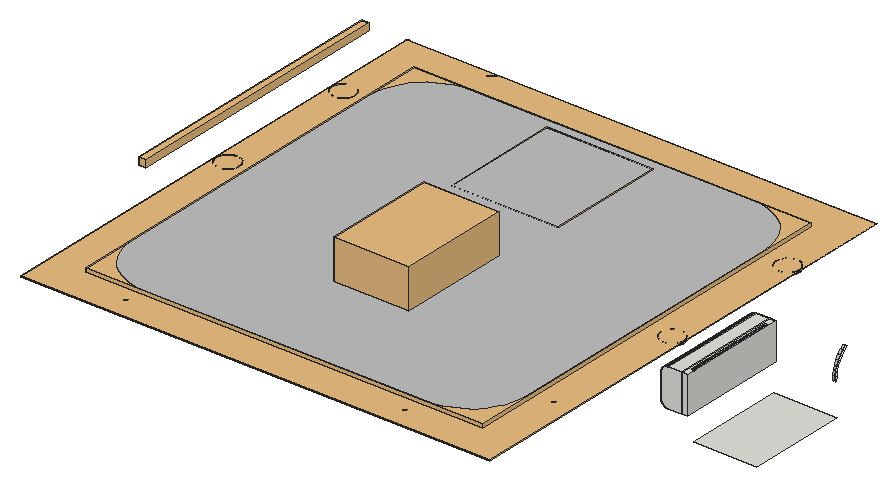
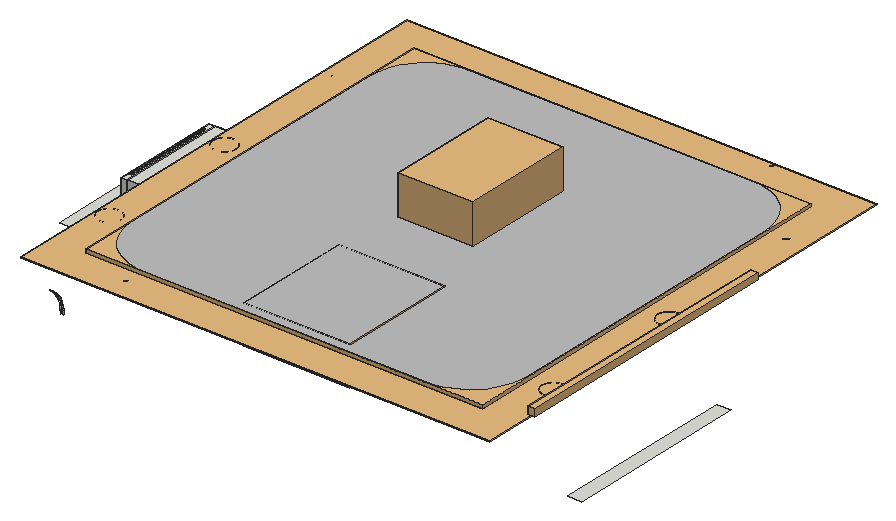
# SketchUp Ruby script. Lengths in inches.
U = 1.inch
M = Sketchup.active_model
def pt(a) = Geom::Point3d.new(a.map { |v| v * U })
def face(e, loops, mat)
  f = e.add_face(loops[0].map { |a| pt(a) })
  loops[1..].each { |l| e.add_face(l.map { |a| pt(a) }).erase! }
  f.material = f.back_material = mat if mat
  f
end
# faces: each face lists its corners as indices into pts; further lists are holes
def faces(e, pts, list, mat = nil) = list.each { |f| face(e, (f[0].is_a?(Array) ? f : [f]).map { |l| l.map { |i| pts[i] } }, mat) }
# xy, xz, yz: faces in a plane at the given z, y or x. An outline is a flat list of corners, or four numbers for a rectangle; further outlines are holes
def ring(l) = l.size == 4 ? [[l[0], l[1]], [l[2], l[1]], [l[2], l[3]], [l[0], l[3]]] : l.each_slice(2).to_a
def flat(e, list, mat, &to3) = list.each { |f| face(e, (f[0].is_a?(Array) ? f : [f]).map { |l| ring(l).map { |u, v| to3.(u, v) } }, mat) }
def xy(e, z, list, mat = nil) = flat(e, list, mat) { |x, y| [x, y, z] }
def xz(e, y, list, mat = nil) = flat(e, list, mat) { |x, z| [x, y, z] }
def yz(e, x, list, mat = nil) = flat(e, list, mat) { |y, z| [x, y, z] }
def lines(e, pts, list) = list.each { |a, b| e.add_line(pt(pts[a]), pt(pts[b])) }
# prism: a flat outline (further loops are holes) pulled along v
def prism(e, loops, v, mat = nil)
  f = face(e, loops, mat); d = Geom::Vector3d.new(v.map { |x| x * U })
  f.pushpull(f.normal.samedirection?(d) ? d.length : -d.length)
end
def box(e, o, s, mat = nil) = prism(e, [[o, [o[0] + s[0], o[1], o[2]], [o[0] + s[0], o[1] + s[1], o[2]], [o[0], o[1] + s[1], o[2]]]], [0, 0, s[2]], mat)
def at(x, y, z, deg = 0) = Geom::Transformation.translation(pt([x, y, z])) * Geom::Transformation.rotation(ORIGIN, Z_AXIS, deg.degrees)
def axes(o, x, y, z) = Geom::Transformation.new([*x, 0, *y, 0, *z, 0, *pt(o).to_a, 1])
def part(name) = M.definitions.add(name)
# library, detail: a bought-in or finely detailed component or shape, given as its bounding box
def library(name, o, s) = part(name).tap { |d| box(d.entities, o, s) }
def detail(e, o, s) = box(e.add_group.entities, o, s)
def put(e, d, t, mat = nil) = e.add_instance(d, t).tap { |i| i.material = mat if mat }
def group(e, t, mat = nil) = e.add_group.tap { |g| g.transformation = t; g.material = mat if mat }.entities
root = M.entities
M.materials.add("[0131_Silver]1").color = [192, 192, 192]
M.materials.add("[Color_004]").color = [142, 142, 142]
M.materials.add("[Color_007]").color = [58, 58, 58]
M.materials.add("[Color_C12]").color = [153, 91, 30]
M.materials.add("[Polished Concrete New]").color = [200, 200, 203]
c1 = library("elliptical+hanging+lamp",[-24.47,-37.92,-16.02],[48.84,73.52,59.72])
c2 = library("Group\#200",[-80.34,-149.03,-93.91],[1.18,2.79,3])
c3 = library("Group\#201",[-80.34,-139.83,-93.89],[1.18,2.84,2.98])
c4 = library("Group\#226",[-0.5,-0.5,0],[173.13,179.13,1.53])
c5 = library("Mesh Light\#5",[-0.5,-0.5,-0.1],[1,1,0.2])
c6 = library("Group\#190",[-80.46,-65.36,-92.6],[1.38,3.58,3.59])
c7 = library("Group\#194",[-88.79,0.67,-41.3125],[0.99,6.14,4.87])
c8 = library("Group\#191",[-88.79,21.34,-41.3125],[0.99,6.53,4.87])
c9 = library("Component\#44",[-0.76,-0.76,-71.54],[3.88,3.88,152.54])
c10 = library("031_FANZART_Zen",[-27.59,-27.12,5.07],[46.53,51.77,17.09])
xy(root,122.28,[[234,631.3,261.625,675.05]])
xy(root,123.47,[[0,635.77,6,717.2]])
xy(root,155.19,[[57.9375,551,54.8,551.2,51.72,551.82,48.75,552.83,45.9375,554.21,43.33,555.96,40.97,558.03,38.9,560.39,37.15,563,35.76,565.8125,34.75,568.79,34.14,571.87,33.9375,575,33.9375,705.125,34.14,708.26,34.75,711.34,35.76,714.3125,37.15,717.125,38.9,719.74,40.97,722.1,43.33,724.17,45.9375,725.91,48.75,727.3,51.72,728.31,54.8,728.92,57.9375,729.125,182.0625,729.125,185.2,728.92,188.28,728.31,191.25,727.3,194.0625,725.91,196.67,724.17,199.03,722.1,201.1,719.74,202.85,717.125,204.24,714.3125,205.25,711.34,205.86,708.26,206.0625,705.125,206.0625,575,205.86,571.87,205.25,568.79,204.24,565.8125,202.85,563,201.1,560.39,199.03,558.03,196.67,555.96,194.0625,554.21,191.25,552.83,188.28,551.82,185.2,551.2,182.0625,551]],"[0131_Silver]1")
yz(root,33.9375,[[575,152.12,705.125,153.65]])
yz(root,206.0625,[[575,152.12,705.125,153.65]],"[0131_Silver]1")
p = [[232.4375,709.3125,111.52],[233.03,709.3125,111.52],[233.03,709.4375,113.41],[232.4375,709.4375,113.41],[234,709.3125,111.52],[234,709.4375,113.41],
  [233.625,709.4375,113.41],[233.625,709.3125,111.52],[233.03,709.81,115.27],[232.4375,709.81,115.27],[234,709.81,115.27],[233.625,709.81,115.27],
  [233.03,710.42,117.07],[232.4375,710.42,117.07],[234,710.42,117.07],[233.625,710.42,117.07],[233.03,711.26,118.77],[232.4375,711.26,118.77],
  [234,711.26,118.77],[233.625,711.26,118.77],[233.03,712.3125,120.35],[232.4375,712.3125,120.35],[234,712.3125,120.35],[233.625,712.3125,120.35],
  [233.03,713.5625,121.78],[232.4375,713.5625,121.78],[234,713.5625,121.78],[233.625,713.5625,121.78],[233.03,714.99,123.03],[232.4375,714.99,123.03],
  [234,714.99,123.03],[233.625,714.99,123.03],[215.71,580.89,152.12],[217,581.0625,152.12],[217,581.0625,153.31],[215.71,580.89,153.31],
  [218.29,580.89,152.12],[218.29,580.89,153.31],[23,635.91,152.12],[21.71,636.09,152.12],[21.71,636.09,153.44],[23,635.91,153.44],
  [24.29,636.09,152.12],[24.29,636.09,153.44],[217,635.91,152.12],[215.71,636.09,152.12],[215.71,636.09,153.31],[217,635.91,153.31],
  [218.29,636.09,152.12],[218.29,636.09,153.31],[20.5,636.58,152.12],[20.5,636.58,153.44],[25.5,636.58,152.12],[25.5,636.58,153.44],
  [214.5,636.58,152.12],[214.5,636.58,153.31],[219.5,636.58,152.12],[219.5,636.58,153.31],[19.46,637.38,152.12],[19.46,637.38,153.44],
  [26.54,637.38,152.12],[26.54,637.38,153.44],[213.46,637.38,152.12],[213.46,637.38,153.31],[220.54,637.38,152.12],[220.54,637.38,153.31],
  [18.67,638.41,152.12],[18.67,638.41,153.44],[27.33,638.41,152.12],[27.33,638.41,153.44],[212.67,638.41,152.12],[212.67,638.41,153.31],
  [221.33,638.41,152.12],[221.33,638.41,153.31],[18.17,639.62,152.12],[18.17,639.62,153.44],[27.83,639.62,152.12],[27.83,639.62,153.44],
  [212.17,639.62,152.12],[212.17,639.62,153.31],[221.83,639.62,152.12],[221.83,639.62,153.31],[18,640.91,152.12],[18,640.91,153.44],
  [28,640.91,152.12],[28,640.91,153.44],[212,640.91,152.12],[212,640.91,153.31],[222,640.91,152.12],[222,640.91,153.31],
  [18.17,642.21,152.12],[18.17,642.21,153.44],[27.83,642.21,152.12],[27.83,642.21,153.44],[212.17,642.21,152.12],[212.17,642.21,153.31],
  [221.83,642.21,152.12],[221.83,642.21,153.31],[18.67,643.41,152.12],[18.67,643.41,153.44],[27.33,643.41,152.12],[27.33,643.41,153.44],
  [212.67,643.41,152.12],[212.67,643.41,153.31],[221.33,643.41,152.12],[221.33,643.41,153.31],[19.46,644.45,152.12],[19.46,644.45,153.44],
  [26.54,644.45,152.12],[26.54,644.45,153.44],[213.46,644.45,152.12],[213.46,644.45,153.31],[220.54,644.45,152.12],[220.54,644.45,153.31],
  [20.5,645.24,152.12],[20.5,645.24,153.44],[25.5,645.24,152.12],[25.5,645.24,153.44],[214.5,645.24,152.12],[214.5,645.24,153.31],
  [219.5,645.24,152.12],[219.5,645.24,153.31],[21.71,645.74,152.12],[21.71,645.74,153.44],[24.29,645.74,152.12],[24.29,645.74,153.44],
  [215.71,645.74,152.12],[215.71,645.74,153.31],[218.29,645.74,152.12],[218.29,645.74,153.31],[23,645.91,152.12],[23,645.91,153.44],
  [217,645.91,152.12],[217,645.91,153.31],[23,699.0625,152.12],[21.71,699.23,152.12],[21.71,699.23,153.44],[23,699.0625,153.44],
  [24.29,699.23,152.12],[24.29,699.23,153.44],[217,699.0625,152.12],[215.71,699.23,152.12],[215.71,699.23,153.31],[217,699.0625,153.31],
  [218.29,699.23,152.12],[218.29,699.23,153.31],[20.5,699.73,152.12],[20.5,699.73,153.44],[25.5,699.73,152.12],[25.5,699.73,153.44],
  [214.5,699.73,152.12],[214.5,699.73,153.31],[219.5,699.73,152.12],[219.5,699.73,153.31],[19.46,700.53,152.12],[19.46,700.53,153.44],
  [26.54,700.53,152.12],[26.54,700.53,153.44],[213.46,700.53,152.12],[213.46,700.53,153.31],[220.54,700.53,152.12],[220.54,700.53,153.31],
  [18.67,701.5625,152.12],[18.67,701.5625,153.44],[27.33,701.5625,152.12],[27.33,701.5625,153.44],[212.67,701.5625,152.12],[212.67,701.5625,153.31],
  [221.33,701.5625,152.12],[221.33,701.5625,153.31],[18.17,702.77,152.12],[18.17,702.77,153.44],[27.83,702.77,152.12],[27.83,702.77,153.44],
  [212.17,702.77,152.12],[212.17,702.77,153.31],[221.83,702.77,152.12],[221.83,702.77,153.31],[18,704.0625,152.12],[18,704.0625,153.44],
  [28,704.0625,152.12],[28,704.0625,153.44],[212,704.0625,152.12],[212,704.0625,153.31],[222,704.0625,152.12],[222,704.0625,153.31],
  [18.17,705.36,152.12],[18.17,705.36,153.44],[27.83,705.36,152.12],[27.83,705.36,153.44],[212.17,705.36,152.12],[212.17,705.36,153.31],
  [221.83,705.36,152.12],[221.83,705.36,153.31],[34.14,708.26,152.12],[34.14,708.26,153.65],[33.9375,705.125,153.65],[33.9375,705.125,152.12],
  [206.0625,705.125,152.12],[206.0625,705.125,153.65],[205.86,708.26,153.65],[205.86,708.26,152.12],[18.67,706.5625,152.12],[18.67,706.5625,153.44],
  [27.33,706.5625,152.12],[27.33,706.5625,153.44],[212.67,706.5625,152.12],[212.67,706.5625,153.31],[221.33,706.5625,152.12],[221.33,706.5625,153.31],
  [19.46,707.6,152.12],[19.46,707.6,153.44],[26.54,707.6,152.12],[26.54,707.6,153.44],[213.46,707.6,152.12],[213.46,707.6,153.31],
  [220.54,707.6,152.12],[220.54,707.6,153.31],[20.5,708.39,152.12],[20.5,708.39,153.44],[25.5,708.39,152.12],[25.5,708.39,153.44],
  [214.5,708.39,152.12],[214.5,708.39,153.31],[219.5,708.39,152.12],[219.5,708.39,153.31],[34.75,711.34,152.12],[34.75,711.34,153.65],
  [205.25,711.34,153.65],[205.25,711.34,152.12],[21.71,708.89,152.12],[21.71,708.89,153.44],[24.29,708.89,152.12],[24.29,708.89,153.44],
  [215.71,708.89,152.12],[215.71,708.89,153.31],[218.29,708.89,152.12],[218.29,708.89,153.31],[23,709.0625,152.12],[23,709.0625,153.44],
  [217,709.0625,152.12],[217,709.0625,153.31],[35.76,714.3125,152.12],[35.76,714.3125,153.65],[204.24,714.3125,153.65],[204.24,714.3125,152.12]]
faces(root,p,[[0,1,2,3],[3,2,8,9],[9,8,12,13],[13,12,16,17],[17,16,20,21],[21,20,24,25],[25,24,28,29]],"[Polished Concrete New]")
faces(root,p,[[4,5,6,7],[5,10,11,6],[10,14,15,11],[14,18,19,15],[18,22,23,19],[22,26,27,23],[26,30,31,27],[32,33,34,35],
  [33,36,37,34],[38,39,40,41],[42,38,41,43],[44,45,46,47],[48,44,47,49],[39,50,51,40],[52,42,43,53],[45,54,55,46],
  [56,48,49,57],[50,58,59,51],[60,52,53,61],[54,62,63,55],[64,56,57,65],[58,66,67,59],[68,60,61,69],[62,70,71,63],
  [72,64,65,73],[66,74,75,67],[76,68,69,77],[70,78,79,71],[80,72,73,81],[74,82,83,75],[84,76,77,85],[78,86,87,79],
  [88,80,81,89],[82,90,91,83],[92,84,85,93],[86,94,95,87],[96,88,89,97],[90,98,99,91],[100,92,93,101],[94,102,103,95],
  [104,96,97,105],[98,106,107,99],[108,100,101,109],[102,110,111,103],[112,104,105,113],[106,114,115,107],[116,108,109,117],[110,118,119,111],
  [120,112,113,121],[114,122,123,115],[124,116,117,125],[118,126,127,119],[128,120,121,129],[122,130,131,123],[130,124,125,131],[126,132,133,127],
  [132,128,129,133],[134,135,136,137],[138,134,137,139],[140,141,142,143],[144,140,143,145],[135,146,147,136],[148,138,139,149],[141,150,151,142],
  [152,144,145,153],[146,154,155,147],[156,148,149,157],[150,158,159,151],[160,152,153,161],[154,162,163,155],[164,156,157,165],[158,166,167,159],
  [168,160,161,169],[162,170,171,163],[172,164,165,173],[166,174,175,167],[176,168,169,177],[170,178,179,171],[180,172,173,181],[174,182,183,175],
  [184,176,177,185],[178,186,187,179],[188,180,181,189],[182,190,191,183],[192,184,185,193],[194,195,196,197],[186,202,203,187],[204,188,189,205],
  [190,206,207,191],[208,192,193,209],[202,210,211,203],[212,204,205,213],[206,214,215,207],[216,208,209,217],[210,218,219,211],[220,212,213,221],
  [214,222,223,215],[224,216,217,225],[226,227,195,194],[218,230,231,219],[232,220,221,233],[222,234,235,223],[236,224,225,237],[230,238,239,231],
  [238,232,233,239],[234,240,241,235],[240,236,237,241],[242,243,227,226]])
faces(root,p,[[198,199,200,201],[201,200,228,229],[229,228,244,245]],"[0131_Silver]1")
put(root,c1,axes([121.33,621.73,143],[0.67,0,0],[0,0.67,0],[0,0,0.67]))
g1 = group(root,at(233.9,652.1,149.98))
prism(g1,[[[-10.63,-19.85,-11.9],[-10.63,-19.78,-12.29],[-10.63,-19.87,-12.29],[-10.63,-19.93,-11.9]]],[0.16,0,0],"[Color_004]")
g2 = group(root,at(233.9,652.1,149.98))
detail(g2,[-10.63,-19.86,-12.43],[0.15,0.1,0.1])
put(root,c2,axes([233.9,652.1,149.98],[0.13234,0,0],[0,0.13234,0],[0,0,0.13234]))
g3 = group(root,at(233.9,652.1,149.98),"[Color_004]")
prism(g3,[[[-10.63,-19.3,-12.03],[-10.63,-19.16,-12.29],[-10.63,-19.1,-12.03],[-10.63,-19.01,-12.03],[-10.63,-19.09,-12.42],[-10.63,-19.1875,-12.42],[-10.63,-19.4,-12.03]]],[0.16,0,0],"[Color_004]")
g4 = group(root,at(233.9,652.1,149.98))
detail(g4,[-10.63,-19.02,-11.99],[0.15,0.09,0.09])
g5 = group(root,at(233.9,652.1,149.98))
prism(g5,[[[-10.63,-18.93,-12.42],[-10.63,-19,-12.03],[-10.63,-18.92,-12.03],[-10.63,-18.85,-12.42]]],[0.16,0,0],"[Color_004]")
g6 = group(root,at(233.9,652.1,149.98))
detail(g6,[-10.63,-18.86,-12.43],[0.15,0.33,0.53])
put(root,c3,axes([233.9,652.1,149.98],[0.13234,0,0],[0,0.13234,0],[0,0,0.13234]))
put(root,c4,at(33.9375,551,153.65))
g7 = group(root,at(18,535.0625,153.31))
xy(g7,0,[[163,0,161.71,0.17,160.5,0.67,159.46,1.46,158.67,2.5,158.17,3.71,158,5,158.17,6.29,158.67,7.5,159.46,8.54,160.5,9.33,161.71,9.83,163,10,164.29,9.83,165.5,9.33,166.54,8.54,167.33,7.5,167.83,6.29,168,5,167.83,3.71,167.33,2.5,166.54,1.46,165.5,0.67,164.29,0.17],[199,36,197.71,36.17,196.5,36.67,195.46,37.46,194.67,38.5,194.17,39.71,194,41,194.17,42.29,194.67,43.5,195.46,44.54,196.5,45.33,197.71,45.83,199,46,200.29,45.83,201.5,45.33,202.54,44.54,203.33,43.5,203.83,42.29,204,41,203.83,39.71,203.33,38.5,202.54,37.46,201.5,36.67,200.29,36.17],[199,100.85,197.71,101.02,196.5,101.52,195.46,102.32,194.67,103.35,194.17,104.56,194,105.85,194.17,107.15,194.67,108.35,195.46,109.39,196.5,110.18,197.71,110.68,199,110.85,200.29,110.68,201.5,110.18,202.54,109.39,203.33,108.35,203.83,107.15,204,105.85,203.83,104.56,203.33,103.35,202.54,102.32,201.5,101.52,200.29,101.02],[199,164,197.71,164.17,196.5,164.67,195.46,165.46,194.67,166.5,194.17,167.71,194,169,194.17,170.29,194.67,171.5,195.46,172.54,196.5,173.33,197.71,173.83,199,174,200.29,173.83,201.5,173.33,202.54,172.54,203.33,171.5,203.83,170.29,204,169,203.83,167.71,203.33,166.5,202.54,165.46,201.5,164.67,200.29,164.17],[163,200,161.71,200.17,160.5,200.67,159.46,201.46,158.67,202.5,158.17,203.71,158,205,158.17,206.29,158.67,207.5,159.46,208.54,160.5,209.33,161.71,209.83,163,210,164.29,209.83,165.5,209.33,166.54,208.54,167.33,207.5,167.83,206.29,168,205,167.83,203.71,167.33,202.5,166.54,201.46,165.5,200.67,164.29,200.17]])
xy(g7,0.125,[[41,0,39.71,0.17,38.5,0.67,37.46,1.46,36.67,2.5,36.17,3.71,36,5,36.17,6.29,36.67,7.5,37.46,8.54,38.5,9.33,39.71,9.83,41,10,42.29,9.83,43.5,9.33,44.54,8.54,45.33,7.5,45.83,6.29,46,5,45.83,3.71,45.33,2.5,44.54,1.46,43.5,0.67,42.29,0.17],[5,36,3.71,36.17,2.5,36.67,1.46,37.46,0.67,38.5,0.17,39.71,0,41,0.17,42.29,0.67,43.5,1.46,44.54,2.5,45.33,3.71,45.83,5,46,6.29,45.83,7.5,45.33,8.54,44.54,9.33,43.5,9.83,42.29,10,41,9.83,39.71,9.33,38.5,8.54,37.46,7.5,36.67,6.29,36.17],[5,100.85,3.71,101.02,2.5,101.52,1.46,102.32,0.67,103.35,0.17,104.56,0,105.85,0.17,107.15,0.67,108.35,1.46,109.39,2.5,110.18,3.71,110.68,5,110.85,6.29,110.68,7.5,110.18,8.54,109.39,9.33,108.35,9.83,107.15,10,105.85,9.83,104.56,9.33,103.35,8.54,102.32,7.5,101.52,6.29,101.02],[5,164,3.71,164.17,2.5,164.67,1.46,165.46,0.67,166.5,0.17,167.71,0,169,0.17,170.29,0.67,171.5,1.46,172.54,2.5,173.33,3.71,173.83,5,174,6.29,173.83,7.5,173.33,8.54,172.54,9.33,171.5,9.83,170.29,10,169,9.83,167.71,9.33,166.5,8.54,165.46,7.5,164.67,6.29,164.17],[41,200,39.71,200.17,38.5,200.67,37.46,201.46,36.67,202.5,36.17,203.71,36,205,36.17,206.29,36.67,207.5,37.46,208.54,38.5,209.33,39.71,209.83,41,210,42.29,209.83,43.5,209.33,44.54,208.54,45.33,207.5,45.83,206.29,46,205,45.83,203.71,45.33,202.5,44.54,201.46,43.5,200.67,42.29,200.17]])
put(g7,c5,axes([102,105,0.0625],[205,0,0],[0,211,0],[0,0,1.125]))
put(root,c6,axes([233.88,652.1,149.98],[0.13234,0,0],[0,0.13234,0],[0,0,0.13234]))
g8 = group(root,at(234,652.1,149.98))
detail(g8,[-11.75,-3.66,-5.47],[0.13,0.83,0.65])
g9 = group(root,at(234,652.1,149.98),"[Color_004]")
prism(g9,[[[-11.62,-1.84,-5.47],[-11.62,-1.63,-5.47],[-11.62,-1.8,-4.82],[-11.62,-2.07,-4.82],[-11.62,-2.21,-5.26],[-11.62,-2.36,-4.82],[-11.62,-2.62,-4.82],[-11.62,-2.78,-5.47],[-11.62,-2.57,-5.47],[-11.62,-2.46,-5.04],[-11.62,-2.33,-5.47],[-11.62,-2.1,-5.47],[-11.62,-1.96,-5.02]]],[-0.13,0,0],"[Color_004]")
g10 = group(root,at(234,652.1,149.98))
prism(g10,[[[-11.62,-1.05,-5.22],[-11.62,-0.98,-5.07],[-11.62,-1.47,-5.07],[-11.62,-1.58,-5.22]]],[-0.13,0,0],"[Color_004]")
g11 = group(root,at(234,652.1,149.98))
detail(g11,[-11.75,-1.58,-5.47],[0.13,0.83,0.65])
g12 = group(root,at(234,652.1,149.98))
prism(g12,[[[-11.62,0.03,-4.98],[-11.62,0.03,-4.82],[-11.62,-0.69,-4.82],[-11.62,-0.69,-4.98],[-11.62,-0.46,-4.98],[-11.62,-0.46,-5.47],[-11.62,-0.22,-5.47],[-11.62,-0.22,-4.98]]],[-0.13,0,0],"[Color_004]")
g13 = group(root,at(234,652.1,149.98))
xy(g13,-16.31,[[-2.61,-24.02,0,24.02]])
xy(g13,-2.9,[[-1.41,-20.07,-1.09,-15.28],[-0.97,-20.07,-0.65,-15.28],[-0.53,-20.07,-0.22,-15.28],[-1.41,-15.02,-1.09,-10.23],[-0.97,-15.02,-0.65,-10.23],
  [-0.53,-15.02,-0.22,-10.23],[-1.41,-9.97,-1.09,-5.18],[-0.97,-9.97,-0.65,-5.18],[-0.53,-9.97,-0.22,-5.18],[-1.41,-4.92,-1.09,-0.13],
  [-0.97,-4.92,-0.65,-0.13],[-0.53,-4.92,-0.22,-0.13],[-1.41,0.13,-1.09,4.92],[-0.97,0.13,-0.65,4.92],[-0.53,0.13,-0.22,4.92],
  [-1.41,5.18,-1.09,9.97],[-0.97,5.18,-0.65,9.97],[-0.53,5.18,-0.22,9.97],[-1.41,10.23,-1.09,15.02],[-0.97,10.23,-0.65,15.02],
  [-0.53,10.23,-0.22,15.02],[-1.41,15.28,-1.09,20.07],[-0.97,15.28,-0.65,20.07],[-0.53,15.28,-0.22,20.07]])
xy(g13,0,[[[-2.61,-24.02,0,24.02],[-1.41,5.18,-1.41,15.02,-1.09,15.02,-1.09,10.23,-1.41,10.23,-1.41,9.97,-1.09,9.97,-1.09,5.18],[-0.53,5.18,-0.53,9.97,-0.22,9.97,-0.22,10.23,-0.53,10.23,-0.53,15.02,-0.22,15.02,-0.22,5.18],[-0.97,15.28,-0.65,20.07],[-0.53,15.28,-0.22,20.07],[-1.41,15.28,-1.09,20.07],[-1.41,-20.07,-1.09,-15.28],[-0.53,-20.07,-0.22,-15.28],[-0.97,-20.07,-0.65,-15.28],[-0.97,5.18,-0.65,9.97],[-0.53,-9.97,-0.22,-5.18],[-0.97,-9.97,-0.65,-5.18],[-1.41,-9.97,-1.09,-5.18],[-0.97,10.23,-0.65,15.02],[-0.97,0.13,-0.65,4.92],[-0.53,0.13,-0.22,4.92],[-1.41,0.13,-1.09,4.92],[-0.53,-15.02,-0.22,-10.23],[-1.41,-15.02,-1.09,-10.23],[-1.41,-4.92,-1.09,-0.13],[-0.97,-4.92,-0.65,-0.13],[-0.53,-4.92,-0.22,-0.13],[-0.97,-15.02,-0.65,-10.23]]])
xz(g13,-24.02,[[-2.61,-16.31,0,0]])
xz(g13,-20.07,[[-1.41,-2.9,-1.09,0],[-0.97,-2.9,-0.65,0],[-0.53,-2.9,-0.22,0]])
xz(g13,-15.28,[[-1.41,-2.9,-1.09,0],[-0.97,-2.9,-0.65,0],[-0.53,-2.9,-0.22,0]])
xz(g13,-15.02,[[-1.41,-2.9,-1.09,0],[-0.97,-2.9,-0.65,0],[-0.53,-2.9,-0.22,0]])
xz(g13,-10.23,[[-1.41,-2.9,-1.09,0],[-0.97,-2.9,-0.65,0],[-0.53,-2.9,-0.22,0]])
xz(g13,-9.97,[[-1.41,-2.9,-1.09,0],[-0.97,-2.9,-0.65,0],[-0.53,-2.9,-0.22,0]])
xz(g13,-5.18,[[-1.41,-2.9,-1.09,0],[-0.97,-2.9,-0.65,0],[-0.53,-2.9,-0.22,0]])
xz(g13,-4.92,[[-1.41,-2.9,-1.09,0],[-0.97,-2.9,-0.65,0],[-0.53,-2.9,-0.22,0]])
xz(g13,-0.13,[[-1.41,-2.9,-1.09,0],[-0.97,-2.9,-0.65,0],[-0.53,-2.9,-0.22,0]])
xz(g13,0.13,[[-1.41,-2.9,-1.09,0],[-0.97,-2.9,-0.65,0],[-0.53,-2.9,-0.22,0]])
xz(g13,4.92,[[-1.41,-2.9,-1.09,0],[-0.97,-2.9,-0.65,0],[-0.53,-2.9,-0.22,0]])
xz(g13,5.18,[[-1.41,-2.9,-1.09,0],[-0.97,-2.9,-0.65,0],[-0.53,-2.9,-0.22,0]])
xz(g13,9.97,[[-1.41,-2.9,-1.09,0],[-0.97,-2.9,-0.65,0],[-0.53,-2.9,-0.22,0]])
xz(g13,10.23,[[-1.41,-2.9,-1.09,0],[-0.97,-2.9,-0.65,0],[-0.53,-2.9,-0.22,0]])
xz(g13,15.02,[[-1.41,-2.9,-1.09,0],[-0.97,-2.9,-0.65,0],[-0.53,-2.9,-0.22,0]])
xz(g13,15.28,[[-1.41,-2.9,-1.09,0],[-0.97,-2.9,-0.65,0],[-0.53,-2.9,-0.22,0]])
xz(g13,20.07,[[-1.41,-2.9,-1.09,0],[-0.97,-2.9,-0.65,0],[-0.53,-2.9,-0.22,0]])
xz(g13,24.02,[[-2.61,-16.31,0,0]])
yz(g13,-2.61,[[-24.02,-16.31,24.02,0]])
yz(g13,-1.41,[[-20.07,-2.9,-15.28,0],[-15.02,-2.9,-10.23,0],[-9.97,-2.9,-5.18,0],[-4.92,-2.9,-0.13,0],[0.13,-2.9,4.92,0],
  [5.18,-2.9,9.97,0],[10.23,-2.9,15.02,0],[15.28,-2.9,20.07,0]])
yz(g13,-1.09,[[-20.07,-2.9,-15.28,0],[-15.02,-2.9,-10.23,0],[-9.97,-2.9,-5.18,0],[-4.92,-2.9,-0.13,0],[0.13,-2.9,4.92,0],
  [5.18,-2.9,9.97,0],[10.23,-2.9,15.02,0],[15.28,-2.9,20.07,0]])
yz(g13,-0.97,[[-20.07,-2.9,-15.28,0],[-15.02,-2.9,-10.23,0],[-9.97,-2.9,-5.18,0],[-4.92,-2.9,-0.13,0],[0.13,-2.9,4.92,0],
  [5.18,-2.9,9.97,0],[10.23,-2.9,15.02,0],[15.28,-2.9,20.07,0]])
yz(g13,-0.65,[[-20.07,-2.9,-15.28,0],[-15.02,-2.9,-10.23,0],[-9.97,-2.9,-5.18,0],[-4.92,-2.9,-0.13,0],[0.13,-2.9,4.92,0],
  [5.18,-2.9,9.97,0],[10.23,-2.9,15.02,0],[15.28,-2.9,20.07,0]])
yz(g13,-0.53,[[-20.07,-2.9,-15.28,0],[-15.02,-2.9,-10.23,0],[-9.97,-2.9,-5.18,0],[-4.92,-2.9,-0.13,0],[0.13,-2.9,4.92,0],
  [5.18,-2.9,9.97,0],[10.23,-2.9,15.02,0],[15.28,-2.9,20.07,0]])
yz(g13,-0.22,[[-20.07,-2.9,-15.28,0],[-15.02,-2.9,-10.23,0],[-9.97,-2.9,-5.18,0],[-4.92,-2.9,-0.13,0],[0.13,-2.9,4.92,0],
  [5.18,-2.9,9.97,0],[10.23,-2.9,15.02,0],[15.28,-2.9,20.07,0]])
yz(g13,0,[[-24.02,-16.31,24.02,0]])
g14 = group(root,at(234,652.1,149.98))
xy(g14,-16.31,[[-8.49,-24.02,-2.61,-20.33],[-8.49,20.33,-2.61,24.02]])
xy(g14,-12.6875,[[-10.58,-20.33,-2.61,20.33]])
xy(g14,-12.43,[[-10.58,-4.46,-10.42,4.46]])
xy(g14,-11.61,[[-10.58,-4.46,-10.42,4.46]])
xy(g14,-11.47,[[-11.62,-24.02,-11.46,-20.33],[-11.46,-20.33,-10.58,20.33],[-11.62,20.33,-11.46,24.02]])
xy(g14,0,[[-8.49,-24.02,-2.61,24.02]])
xz(g14,-24.02,[[-8.49,-16.31,-2.61,-16.31,-2.61,0,-8.49,0,-8.49,-0.16,-8.96,-0.19,-9.41,-0.3,-9.84,-0.48,-10.24,-0.72,-10.59,-1.03,-10.9,-1.38,-11.14,-1.78,-11.32,-2.21,-11.43,-2.66,-11.46,-3.125,-11.46,-11.47,-11.62,-11.47,-11.62,-13.18,-11.58,-13.67,-11.47,-14.15,-11.28,-14.6,-11.02,-15.02,-10.7,-15.39,-10.33,-15.71,-9.91,-15.97,-9.46,-16.16,-8.98,-16.27]])
xz(g14,-20.33,[[-8.49,-16.31,-8.98,-16.27,-9.46,-16.16,-9.91,-15.97,-10.33,-15.71,-10.7,-15.39,-11.02,-15.02,-11.28,-14.6,-11.47,-14.15,-11.58,-13.67,-11.62,-13.18,-11.62,-11.47,-10.58,-11.47,-10.58,-12.6875,-2.61,-12.6875,-2.61,-16.31]])
xz(g14,-4.46,[[-10.58,-12.43,-10.42,-11.61]])
xz(g14,4.46,[[-10.58,-12.43,-10.42,-11.61]])
xz(g14,20.33,[[-8.49,-16.31,-2.61,-16.31,-2.61,-12.6875,-10.58,-12.6875,-10.58,-11.47,-11.62,-11.47,-11.62,-13.18,-11.58,-13.67,-11.47,-14.15,-11.28,-14.6,-11.02,-15.02,-10.7,-15.39,-10.33,-15.71,-9.91,-15.97,-9.46,-16.16,-8.98,-16.27]])
xz(g14,24.02,[[-8.49,-16.31,-8.98,-16.27,-9.46,-16.16,-9.91,-15.97,-10.33,-15.71,-10.7,-15.39,-11.02,-15.02,-11.28,-14.6,-11.47,-14.15,-11.58,-13.67,-11.62,-13.18,-11.62,-11.47,-11.46,-11.47,-11.46,-3.125,-11.43,-2.66,-11.32,-2.21,-11.14,-1.78,-10.9,-1.38,-10.59,-1.03,-10.24,-0.72,-9.84,-0.48,-9.41,-0.3,-8.96,-0.19,-8.49,-0.16,-8.49,0,-2.61,0,-2.61,-16.31]])
yz(g14,-11.62,[[-24.02,-13.18,-20.33,-11.47],[20.33,-13.18,24.02,-11.47]])
yz(g14,-11.46,[[-24.02,-11.47,24.02,-3.125]])
yz(g14,-10.58,[[[-20.33,-12.6875,20.33,-11.47],[-4.46,-12.43,4.46,-11.61]]])
yz(g14,-10.42,[[-4.46,-12.43,4.46,-11.61]],"[Color_007]")
yz(g14,-8.49,[[-24.02,-0.16,24.02,0]])
yz(g14,-2.61,[[-24.02,-16.31,-20.33,-16.31,-20.33,-12.6875,20.33,-12.6875,20.33,-16.31,24.02,-16.31,24.02,0,-24.02,0]])
p = [[-9.46,-24.02,-16.16],[-9.46,-20.33,-16.16],[-8.98,-20.33,-16.27],[-8.98,-24.02,-16.27],[-8.49,-20.33,-16.31],[-8.49,-24.02,-16.31],
  [-9.46,20.33,-16.16],[-9.46,24.02,-16.16],[-8.98,24.02,-16.27],[-8.98,20.33,-16.27],[-8.49,24.02,-16.31],[-8.49,20.33,-16.31],
  [-9.91,-20.33,-15.97],[-9.91,-24.02,-15.97],[-9.91,20.33,-15.97],[-9.91,24.02,-15.97],[-10.33,-24.02,-15.71],[-10.33,-20.33,-15.71],
  [-10.33,20.33,-15.71],[-10.33,24.02,-15.71],[-10.7,-24.02,-15.39],[-10.7,-20.33,-15.39],[-10.7,20.33,-15.39],[-10.7,24.02,-15.39],
  [-11.02,-24.02,-15.02],[-11.02,-20.33,-15.02],[-11.02,20.33,-15.02],[-11.02,24.02,-15.02],[-11.28,-24.02,-14.6],[-11.28,-20.33,-14.6],
  [-11.28,20.33,-14.6],[-11.28,24.02,-14.6],[-11.47,-20.33,-14.15],[-11.47,-24.02,-14.15],[-11.47,20.33,-14.15],[-11.47,24.02,-14.15],
  [-11.58,-24.02,-13.67],[-11.58,-20.33,-13.67],[-11.58,20.33,-13.67],[-11.58,24.02,-13.67],[-11.62,-24.02,-13.18],[-11.62,-20.33,-13.18],
  [-11.62,20.33,-13.18],[-11.62,24.02,-13.18],[-11.46,24.02,-3.125],[-11.46,-24.02,-3.125],[-11.43,-24.02,-2.66],[-11.43,24.02,-2.66],
  [-11.32,-24.02,-2.21],[-11.32,24.02,-2.21],[-11.14,24.02,-1.78],[-11.14,-24.02,-1.78],[-10.9,-24.02,-1.38],[-10.9,24.02,-1.38],
  [-10.59,-24.02,-1.03],[-10.59,24.02,-1.03],[-10.24,-24.02,-0.72],[-10.24,24.02,-0.72],[-9.84,-24.02,-0.48],[-9.84,24.02,-0.48],
  [-9.41,24.02,-0.3],[-9.41,-24.02,-0.3],[-8.96,-24.02,-0.19],[-8.96,24.02,-0.19],[-8.49,-24.02,-0.16],[-8.49,24.02,-0.16]]
faces(g14,p,[[0,1,2,3],[4,5,3,2],[6,7,8,9],[10,11,9,8],[12,1,0,13],[6,14,15,7],[12,13,16,17],[15,14,18,19],
  [20,21,17,16],[22,23,19,18],[21,20,24,25],[23,22,26,27],[28,29,25,24],[30,31,27,26],[32,29,28,33],[30,34,35,31],
  [32,33,36,37],[35,34,38,39],[40,41,37,36],[42,43,39,38],[44,45,46,47],[48,49,47,46],[50,49,48,51],[50,51,52,53],
  [54,55,53,52],[55,54,56,57],[58,59,57,56],[60,59,58,61],[60,61,62,63],[64,65,63,62]])
g15 = group(root,at(234,652.1,149.98))
prism(g15,[[[-11.62,23.99,-11.47],[-11.62,23.99,-3.125],[-11.58,23.99,-2.64],[-11.47,23.99,-2.16],[-11.28,23.99,-1.71],[-11.02,23.99,-1.29],[-10.7,23.99,-0.92],[-10.33,23.99,-0.6],[-9.91,23.99,-0.34],[-9.46,23.99,-0.15],[-8.98,23.99,-0.04],[-8.49,23.99,0],[-8.49,23.99,-0.16],[-8.96,23.99,-0.19],[-9.41,23.99,-0.3],[-9.84,23.99,-0.48],[-10.24,23.99,-0.72],[-10.59,23.99,-1.03],[-10.9,23.99,-1.38],[-11.14,23.99,-1.78],[-11.32,23.99,-2.21],[-11.43,23.99,-2.66],[-11.46,23.99,-3.125],[-11.46,23.99,-11.47]]],[0,-47.98,0])
g16 = group(root,at(234,652.1,149.98))
xy(g16,-15.84,[[-8.4,-20.33,-5.52,20.33]])
xy(g16,-13.34,[[-10.9,-20.33,-10.53,-11.65],[-10.9,-11.33,-10.53,6.03],[-10.9,6.34,-10.53,20.33]])
xy(g16,-12.6875,[[-10.53,-20.33,-5.52,-20.33,-5.52,20.33,-10.53,20.33,-10.53,6.34,-10.9,6.34,-10.9,6.03,-10.53,6.03,-10.53,-11.33,-10.9,-11.33,-10.9,-11.65,-10.53,-11.65]])
xz(g16,-20.33,[[-8.4,-15.84,-5.52,-15.84,-5.52,-12.6875,-10.53,-12.6875,-10.53,-13.34,-10.9,-13.34,-10.89,-13.39,-10.87,-13.73,-10.78,-14.12,-10.625,-14.48,-10.42,-14.8125,-10.17,-15.11,-9.87,-15.37,-9.53,-15.57,-9.17,-15.72,-8.79,-15.8125]])
xz(g16,-11.65,[[-10.9,-13.34,-10.53,-12.6875]])
xz(g16,-11.33,[[-10.9,-13.34,-10.53,-12.6875]])
xz(g16,6.03,[[-10.9,-13.34,-10.53,-12.6875]])
xz(g16,6.34,[[-10.9,-13.34,-10.53,-12.6875]])
xz(g16,20.33,[[-8.4,-15.84,-8.79,-15.8125,-9.17,-15.72,-9.53,-15.57,-9.87,-15.37,-10.17,-15.11,-10.42,-14.8125,-10.625,-14.48,-10.78,-14.12,-10.87,-13.73,-10.89,-13.39,-10.9,-13.34,-10.53,-13.34,-10.53,-12.6875,-5.52,-12.6875,-5.52,-15.84]])
yz(g16,-10.9,[[-11.65,-13.34,-11.33,-12.6875],[6.03,-13.34,6.34,-12.6875]])
yz(g16,-10.53,[[-20.33,-13.34,-11.65,-12.6875],[-11.33,-13.34,6.03,-12.6875],[6.34,-13.34,20.33,-12.6875]],"[Color_007]")
yz(g16,-5.52,[[-20.33,-15.84,20.33,-12.6875]])
p = [[-9.17,-20.33,-15.72],[-9.17,20.33,-15.72],[-8.79,20.33,-15.8125],[-8.79,-20.33,-15.8125],[-8.4,20.33,-15.84],[-8.4,-20.33,-15.84],
  [-9.53,20.33,-15.57],[-9.53,-20.33,-15.57],[-9.87,-20.33,-15.37],[-9.87,20.33,-15.37],[-10.17,-20.33,-15.11],[-10.17,20.33,-15.11],
  [-10.42,-20.33,-14.8125],[-10.42,20.33,-14.8125],[-10.625,-20.33,-14.48],[-10.625,20.33,-14.48],[-10.78,20.33,-14.12],[-10.78,-20.33,-14.12],
  [-10.87,-20.33,-13.73],[-10.87,20.33,-13.73],[-10.89,-20.33,-13.39],[-10.89,-11.65,-13.39],[-10.89,-11.33,-13.39],[-10.89,6.03,-13.39],
  [-10.89,6.34,-13.39],[-10.89,20.33,-13.39],[-10.9,20.33,-13.34],[-10.9,-20.33,-13.34],[-10.9,-11.65,-13.34],[-10.9,-11.33,-13.34],
  [-10.9,6.03,-13.34],[-10.9,6.34,-13.34]]
faces(g16,p,[[0,1,2,3],[4,5,3,2],[6,1,0,7],[6,7,8,9],[10,11,9,8],[11,10,12,13],[14,15,13,12],[16,15,14,17],
  [16,17,18,19],[18,20,21,22,23,24,25,19]])
faces(g16,p,[[26,25,24,23,22,21,20,27,28,29,30,31]],"[Color_C12]")
put(root,c7,axes([234,652.1,149.98],[0.13234,0,0],[0,0.13234,0],[0,0,0.13234]))
g17 = group(root,at(234,652.1,149.98))
prism(g17,[[[-11.62,1.66,-5.47],[-11.62,1.9,-5.47],[-11.62,1.55,-4.86],[-11.62,1.54,-4.85],[-11.62,1.53,-4.84],[-11.62,1.52,-4.83],[-11.62,1.51,-4.82],[-11.62,1.49,-4.82],[-11.62,1.33,-4.82],[-11.62,1.32,-4.82],[-11.62,1.3,-4.83],[-11.62,1.29,-4.84],[-11.62,1.28,-4.85],[-11.62,1.27,-4.86],[-11.62,0.92,-5.47],[-11.62,1.16,-5.47],[-11.62,1.24,-5.33],[-11.62,1.59,-5.33]],[[-11.62,1.52,-5.22],[-11.62,1.3,-5.22],[-11.62,1.41,-5.03]]],[-0.13,0,0],"[Color_004]")
g18 = group(root,at(234,652.1,149.98))
detail(g18,[-11.75,1.87,-5.47],[0.13,0.86,0.65])
put(root,c8,axes([234,652.1,149.98],[0.13234,0,0],[0,0.13234,0],[0,0,0.13234]))
put(root,c9,axes([8.86,667.82,162.89],[0,0,-0.798],[0.798,0,0],[0,0.798,0]))
put(root,c10,at(122.375,700.5,133.02))
